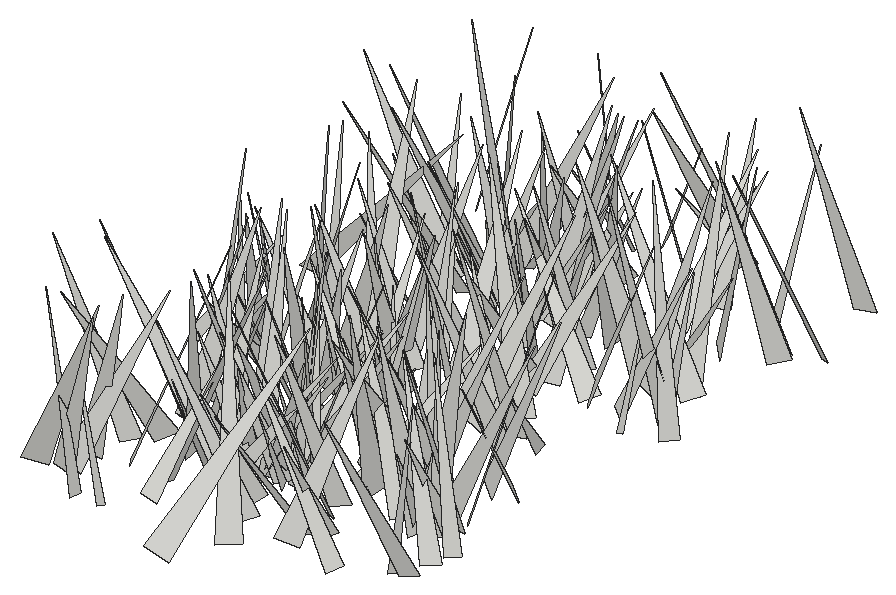
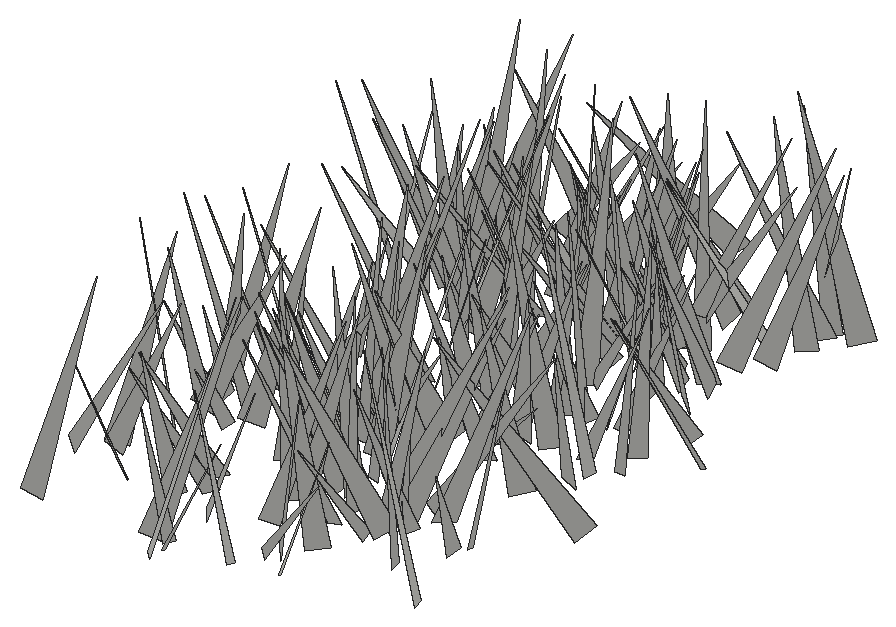
# SketchUp Ruby script. Lengths in inches.
U = 1.inch
M = Sketchup.active_model
def pt(a) = Geom::Point3d.new(a.map { |v| v * U })
def face(e, loops, mat)
  f = e.add_face(loops[0].map { |a| pt(a) })
  loops[1..].each { |l| e.add_face(l.map { |a| pt(a) }).erase! }
  f.material = f.back_material = mat if mat
  f
end
# faces: each face lists its corners as indices into pts; further lists are holes
def faces(e, pts, list, mat = nil) = list.each { |f| face(e, (f[0].is_a?(Array) ? f : [f]).map { |l| l.map { |i| pts[i] } }, mat) }
# xy, xz, yz: faces in a plane at the given z, y or x. An outline is a flat list of corners, or four numbers for a rectangle; further outlines are holes
def ring(l) = l.size == 4 ? [[l[0], l[1]], [l[2], l[1]], [l[2], l[3]], [l[0], l[3]]] : l.each_slice(2).to_a
def flat(e, list, mat, &to3) = list.each { |f| face(e, (f[0].is_a?(Array) ? f : [f]).map { |l| ring(l).map { |u, v| to3.(u, v) } }, mat) }
def xy(e, z, list, mat = nil) = flat(e, list, mat) { |x, y| [x, y, z] }
def xz(e, y, list, mat = nil) = flat(e, list, mat) { |x, z| [x, y, z] }
def yz(e, x, list, mat = nil) = flat(e, list, mat) { |y, z| [x, y, z] }
def lines(e, pts, list) = list.each { |a, b| e.add_line(pt(pts[a]), pt(pts[b])) }
# prism: a flat outline (further loops are holes) pulled along v
def prism(e, loops, v, mat = nil)
  f = face(e, loops, mat); d = Geom::Vector3d.new(v.map { |x| x * U })
  f.pushpull(f.normal.samedirection?(d) ? d.length : -d.length)
end
def box(e, o, s, mat = nil) = prism(e, [[o, [o[0] + s[0], o[1], o[2]], [o[0] + s[0], o[1] + s[1], o[2]], [o[0], o[1] + s[1], o[2]]]], [0, 0, s[2]], mat)
def at(x, y, z, deg = 0) = Geom::Transformation.translation(pt([x, y, z])) * Geom::Transformation.rotation(ORIGIN, Z_AXIS, deg.degrees)
def axes(o, x, y, z) = Geom::Transformation.new([*x, 0, *y, 0, *z, 0, *pt(o).to_a, 1])
def part(name) = M.definitions.add(name)
# library, detail: a bought-in or finely detailed component or shape, given as its bounding box
def library(name, o, s) = part(name).tap { |d| box(d.entities, o, s) }
def detail(e, o, s) = box(e.add_group.entities, o, s)
def put(e, d, t, mat = nil) = e.add_instance(d, t).tap { |i| i.material = mat if mat }
def group(e, t, mat = nil) = e.add_group.tap { |g| g.transformation = t; g.material = mat if mat }.entities
root = M.entities
c1 = part("fur_instance\#9")
p = [[0.8125,0,1.79],[0.67,-0.02,1.48],[0,-0.11,0],[0,0.11,0]]
faces(c1.entities,p,[[0,1,2,3]])
put(root,c1,axes([478.11,318.66,-21.66],[1.0703,-6.74535,2.51722],[-6.58595,-1.94546,-2.41292],[-2.90886,1.9228,6.3893]))
put(root,c1,axes([473.07,330.8,-21.66],[3.04424,4.32162,0.01521],[3.85535,-2.70735,-2.39804],[1.95268,-1.39208,4.71097]))
put(root,c1,axes([478.31,348.03,-21.66],[-4.48023,1.71415,0.10108],[1.53614,4.12726,-1.90446],[0.76734,1.74596,4.4027]))
put(root,c1,axes([478.21,337.2,-21.66],[1.19098,5.93826,0.851],[5.76454,-1.37303,1.51343],[-1.66049,-0.50738,5.86438]))
put(root,c1,axes([476.59,334.39,-21.66],[-1.94792,-5.41513,0.85515],[-5.11405,2.12183,1.78705],[1.97517,0.15336,5.47032]))
put(root,c1,axes([479.69,311.34,-21.66],[-6.30755,-1.0303,0.95825],[-1.23667,6.15876,-1.51833],[0.67114,1.66527,6.20817]))
put(root,c1,axes([479.28,334.33,-21.66],[-4.32688,2.05759,1.06704],[2.30248,4.07514,1.47851],[0.2661,-1.80382,4.55737]))
put(root,c1,axes([477.84,347.04,-21.66],[-4.12038,-2.11418,1.50488],[-1.47976,4.23386,1.89649],[2.13184,-1.14743,4.225]))
put(root,c1,axes([478.76,325.4,-21.66],[4.06044,6.49572,1.60929],[6.19974,-4.35997,1.95581],[-2.5194,-0.26008,7.4065]))
put(root,c1,axes([476.96,332.22,-21.66],[6.03542,-2.39463,0.80521],[-2.12324,-5.9379,-1.74415],[-1.3691,-1.34759,6.25448]))
put(root,c1,axes([475.61,328.35,-21.66],[3.92135,-2.35365,0.03406],[-2.05535,-3.39138,2.27856],[1.14733,1.96892,3.96545]))
put(root,c1,axes([473.56,341.38,-21.66],[6.0984,-4.54505,0.22334],[-3.82324,-4.91501,4.37303],[2.46783,3.61705,6.22291]))
put(root,c1,axes([479.55,320.28,-21.66],[4.2838,-6.03866,0.74714],[-5.20831,-4.11147,-3.36808],[-3.14598,-1.41597,6.59337]))
put(root,c1,axes([475.19,313.07,-21.66],[4.73655,-6.32836,0.37656],[-6.13582,-4.45802,2.25891],[1.59428,1.644,7.57499]))
put(root,c1,axes([481.02,345.5,-21.66],[-7.69272,2.37823,1.5322],[2.71051,7.46743,2.01798],[0.8104,-2.40066,7.79498]))
put(root,c1,axes([481.03,329.86,-21.66],[-5.46466,-2.11839,0.66349],[-2.21236,5.05235,-2.09036],[-0.18243,2.18553,5.47545]))
put(root,c1,axes([482.32,344.96,-21.66],[-2.35699,-6.63901,0.53799],[-6.01099,1.87426,-3.2057],[-2.86948,1.52709,6.27339]))
put(root,c1,axes([476.08,354.2,-21.66],[7.20484,3.15988,1.15153],[3.35999,-6.88107,-2.14053],[-0.14588,-2.42624,7.57051]))
put(root,c1,axes([478.59,323.08,-21.66],[5.94248,2.0649,1.47313],[1.51819,-5.90154,2.14801],[-2.032,1.62942,5.91295]))
put(root,c1,axes([481.06,325.37,-21.66],[-6.67208,0.88571,0.68005],[0.61302,6.34873,-2.25421],[0.93335,2.16166,6.3419]))
put(root,c1,axes([477.25,313.28,-21.66],[0.83878,-6.84447,1.51714],[-6.71971,-0.34936,2.13903],[1.99848,1.69801,6.55552]))
put(root,c1,axes([477.18,315.86,-21.66],[2.07111,-6.85146,1.31632],[-6.80663,-1.68294,1.94991],[1.53132,1.78604,6.88693]))
put(root,c1,axes([484.07,318.57,-21.66],[-5.6206,-6.05261,0.8091],[-5.56666,4.62654,-4.06048],[-2.5102,3.29256,7.1929]))
put(root,c1,axes([479.79,330.34,-21.66],[4.40481,-2.70951,0.82389],[-1.71706,-3.76665,-3.20728],[-2.2521,-2.42766,4.05674]))
put(root,c1,axes([479.56,339.92,-21.66],[-4.86903,5.31705,1.90275],[5.12727,5.21523,-1.45307],[2.36698,-0.35954,7.06166]))
put(root,c1,axes([481.65,311.35,-21.66],[-4.16837,-0.36819,0.02902],[-0.35612,3.91965,-1.4217],[-0.09791,1.41863,3.93569]))
put(root,c1,axes([477.19,313.99,-21.66],[0.42432,7.03314,2.02201],[6.63788,0.48281,-3.07232],[3.08094,-2.00885,6.34082]))
put(root,c1,axes([483.37,320.27,-21.66],[-7.87957,1.88276,1.17896],[2.17634,7.41366,2.70618],[0.44527,-2.91806,7.63603]))
put(root,c1,axes([480.29,323.67,-21.66],[4.99403,0.89918,1.35491],[0.3935,-4.91429,1.81096],[-1.5778,1.62046,4.74018]))
put(root,c1,axes([477.8125,335.72,-21.66],[8.03575,1.73258,0.69022],[1.85682,-7.7181,-2.24381],[-0.17451,-2.34107,7.90825]))
put(root,c1,axes([483.51,348.08,-21.66],[1.68916,7.29229,2.94864],[7.0223,-2.75681,2.79508],[-3.5439,-1.98689,6.94394]))
put(root,c1,axes([479.83,316.42,-21.66],[6.02604,4.35688,0.13616],[4.14402,-5.7981,2.12678],[-1.35204,1.64734,7.12547]))
put(root,c1,axes([479.25,322.59,-21.66],[0.24663,7.62872,2.41582],[7.70784,0.42293,-2.12242],[2.15005,-2.39126,7.33168]))
put(root,c1,axes([483.25,346.38,-21.66],[0.03934,-7.1777,0.79174],[-6.87762,-0.27857,-2.18369],[-2.20103,0.74216,6.83757]))
put(root,c1,axes([480,351.46,-21.66],[6.17791,2.14602,1.95241],[2.61385,-6.11017,-1.55482],[-1.25898,-2.15507,6.35252]))
put(root,c1,axes([484.52,339.01,-21.66],[-3.03964,-3.22245,0.08473],[-2.53096,2.3136,-2.80576],[-1.9964,1.97328,3.42802]))
put(root,c1,axes([484.83,345.3,-21.66],[-3.02685,-7.70536,1.30124],[-7.48247,2.45538,-2.86554],[-2.25353,2.19686,7.76679]))
put(root,c1,axes([482.19,330.73,-21.66],[-7.10447,-2.39928,3.44832],[-3.25719,7.42464,-1.54476],[2.65295,2.69055,7.33783]))
put(root,c1,axes([483.21,323.52,-21.66],[0.69074,-4.72184,2.34998],[-4.89788,-1.45354,-1.48096],[-1.95676,1.97148,4.53648]))
put(root,c1,axes([481.4,322.3,-21.66],[4.67368,1.9817,0.84614],[1.46066,-4.3994,2.23565],[-1.58416,1.79011,4.55767]))
put(root,c1,axes([483.39,321.68,-21.66],[0.65103,4.23875,0.31259],[3.78552,-0.72206,1.9071],[-1.9325,0.01355,3.84107]))
put(root,c1,axes([484.04,334.5625,-21.66],[-0.66678,7.09806,0.59701],[6.83624,0.46921,2.05647],[-2.00116,-0.76214,6.82627]))
put(root,c1,axes([484.17,322.98,-21.66],[-2.33068,3.85921,0.35584],[3.66264,2.05758,1.6744],[-1.26695,-1.15111,4.18592]))
put(root,c1,axes([484.62,326.82,-21.66],[-2.52034,-4.28654,0.32351],[-4.12689,2.30776,-1.57296],[-1.20326,1.06349,4.71724]))
put(root,c1,axes([481.94,330.58,-21.66],[4.14579,-2.60609,2.17076],[-3.31381,-3.84297,1.71517],[-0.72292,2.67047,4.58667]))
put(root,c1,axes([484.58,333.97,-21.66],[-5.48359,2.23586,1.70204],[2.68404,5.27249,1.72124],[0.83185,-2.27324,5.66623]))
put(root,c1,axes([483.26,320.5,-21.66],[-5.22484,3.83291,1.4033],[3.4058,5.3502,-1.93269],[2.24967,0.80218,6.18505]))
put(root,c1,axes([484.76,322.68,-21.66],[-1.35927,-4.19334,1.10265],[-4.18909,0.97193,-1.4678],[-1.11869,1.45561,4.1566]))
put(root,c1,axes([483.79,323.89,-21.66],[-5.87667,-3.9224,1.1719],[-3.54254,5.90008,1.98324],[2.05159,-1.04767,6.78139]))
put(root,c1,axes([486.01,335.86,-21.66],[-1.67581,5.69721,1.32161],[5.39716,0.9769,2.63242],[-2.25291,-1.89755,5.32325]))
put(root,c1,axes([482.33,347.89,-21.66],[3.64505,-0.39812,0.27738],[-0.20845,-3.18305,-1.82936],[-0.43816,-1.79764,3.17779]))
put(root,c1,axes([481.97,319.91,-21.66],[7.49694,-1.26912,1.50095],[-0.87324,-7.45265,-1.93987],[-1.76095,-1.70734,7.35199]))
put(root,c1,axes([483.36,323.23,-21.66],[4.16098,5.56887,0.17793],[5.30628,-4.02846,1.99315],[-1.69922,1.05685,6.65984]))
put(root,c1,axes([485.13,321.75,-21.66],[-7.34828,2.49323,1.09592],[2.03506,7.1224,-2.5582],[1.80991,2.11416,7.32591]))
put(root,c1,axes([481.69,334.51,-21.66],[3.71453,-6.09838,0.78607],[-6.05056,-3.46164,1.73599],[1.09493,1.55972,6.92635]))
put(root,c1,axes([484.27,331.06,-21.66],[6.50516,0.09741,3.11354],[0.81371,-7.01185,-1.48071],[-3.00691,-1.68675,6.33514]))
put(root,c1,axes([481.875,347.5625,-21.66],[2.63596,-3.80697,0.02165],[-3.40971,-2.34911,2.07299],[1.69332,1.196,4.14053]))
put(root,c1,axes([483.36,313.79,-21.66],[-0.37436,5.47936,0.25355],[5.20879,0.43477,-1.70506],[1.71934,-0.12411,5.22075]))
put(root,c1,axes([487.06,355.18,-21.66],[-2.6027,-3.00196,0.39616],[-2.70686,2.07255,-2.07851],[-1.35707,1.62343,3.38609]))
put(root,c1,axes([484.69,356.57,-21.66],[-2.93741,-3.09466,0.01129],[-2.71699,2.58635,2.03327],[1.48156,-1.39259,3.75115]))
put(root,c1,axes([486.47,339.98,-21.66],[1.14957,-5.99203,1.40359],[-5.68779,-1.57972,-2.08556],[-2.35023,0.89221,5.73379]))
put(root,c1,axes([483.59,349.69,-21.66],[3.8069,0.05751,0.20355],[-0.0416,-3.39391,1.73693],[-0.20739,1.73647,3.38805]))
put(root,c1,axes([483.33,330.68,-21.66],[0.81031,-5.69395,0.84212],[-5.55553,-0.55126,1.61834],[1.50543,1.03047,5.51893]))
put(root,c1,axes([486.34,354.46,-21.66],[3.70498,4.05955,2.96614],[3.93602,-4.63444,1.42637],[-3.1282,-1.02317,5.30776]))
put(root,c1,axes([482.92,348.75,-21.66],[6.18283,-3.26103,2.17206],[-3.91127,-5.37775,3.05962],[-0.2327,3.74499,6.28493]))
put(root,c1,axes([486.83,320.23,-21.66],[-7.37463,3.18086,0.67882],[2.84062,7.11825,-2.49505],[1.58417,2.04365,7.63399]))
put(root,c1,axes([486.42,319.71,-21.66],[-4.94323,1.53486,1.76986],[2.06825,4.80019,1.61379],[1.10026,-2.12747,4.91803]))
put(root,c1,axes([483.8,338.05,-21.66],[-0.17372,7.00266,1.70424],[6.95108,0.61311,-1.81067],[1.90374,-1.5996,6.76675]))
put(root,c1,axes([482.94,315.8125,-21.66],[8.11647,0.24258,0.67526],[0.10402,-7.98511,1.61836],[-0.70993,1.60345,7.95719]))
put(root,c1,axes([486.96,336.92,-21.66],[-5.33411,1.7362,0.45715],[1.45522,5.02033,-2.08679],[1.05153,1.85957,5.20696]))
put(root,c1,axes([489.61,315.59,-21.66],[-2.20634,6.02099,1.75888],[5.48729,0.94934,3.63349],[-3.03901,-2.65713,5.28374]))
put(root,c1,axes([484.9,327.28,-21.66],[7.37439,-3.31849,1.28024],[-2.90244,-7.31769,-2.24953],[-2.05603,-1.57231,7.76747]))
put(root,c1,axes([486.43,330.4,-21.66],[-4.56686,4.07542,0.09193],[3.68922,4.19072,-2.51023],[1.73411,1.8173,5.58247]))
put(root,c1,axes([489.04,327.64,-21.66],[-3.06534,4.86368,0.18481],[4.51167,2.75744,2.26433],[-1.82603,-1.35165,5.28436]))
put(root,c1,axes([485.68,320.78,-21.66],[4.75134,-2.11282,0.36953],[-1.90852,-4.57438,-1.61505],[-0.97883,-1.33672,4.94275]))
put(root,c1,axes([487.5,343.29,-21.66],[-5.6893,-5.57398,0.54513],[-5.22917,5.56506,2.3282],[2.00554,-1.30211,7.61688]))
put(root,c1,axes([488.46,330.03,-21.66],[-5.41908,-0.82486,1.13145],[-1.12996,5.24719,-1.58656],[0.82691,1.76453,5.24687]))
put(root,c1,axes([484.43,336.04,-21.66],[3.61715,-5.66391,0.01487],[-5.50634,-3.51236,1.58351],[1.3268,0.86448,6.53117]))
put(root,c1,axes([486.05,348.05,-21.66],[6.38697,0.74513,2.00431],[1.2691,-6.40204,-1.66407],[-1.72101,-1.95564,6.21124]))
put(root,c1,axes([488.38,320.35,-21.66],[2.87814,-5.28951,1.31735],[-4.95416,-3.15966,-1.86304],[-2.27391,0.18887,5.72641]))
put(root,c1,axes([486.94,322.74,-21.66],[5.11337,-4.37567,0.02712],[-4.08728,-4.79107,-2.37351],[-1.56248,-1.78687,6.29758]))
put(root,c1,axes([489.11,341.85,-21.66],[1.07794,-7.21694,3.00432],[-7.53412,-1.768,-1.54384],[-2.08502,2.65746,7.13181]))
put(root,c1,axes([490.07,340.4,-21.66],[-2.15609,-3.98258,0.83043],[-3.73233,1.56246,-2.1972],[-1.61872,1.70208,3.96005]))
put(root,c1,axes([484.88,352.75,-21.66],[3.43044,-6.71204,0.2285],[-6.5076,-3.25868,1.97581],[1.6598,1.09595,7.27431]))
put(root,c1,axes([485.15,324.07,-21.66],[4.61387,-2.10989,0.31356],[-1.93342,-3.82099,2.73855],[0.90102,2.60502,4.2708]))
put(root,c1,axes([488.56,317.84,-21.66],[3.46257,-3.0651,1.27719],[-2.41097,-3.5895,-2.07802],[-2.28326,-0.85797,4.13111]))
put(root,c1,axes([489.51,348.25,-21.66],[0.21483,-6.37799,2.26736],[-6.52313,-0.80094,-1.63496],[-1.80789,2.13204,6.16862]))
put(root,c1,axes([488.94,336.27,-21.66],[-6.13074,4.86156,0.06985],[4.48302,5.69573,-2.94734],[1.88206,2.26926,7.24803]))
put(root,c1,axes([487.48,333.01,-21.66],[7.10031,-2.91459,1.55919],[-2.29482,-7.00551,-2.64516],[-2.37902,-1.94118,7.20502]))
put(root,c1,axes([486.01,349.71,-21.66],[1.82211,6.46965,0.85286],[6.26515,-1.48669,-2.10749],[1.8253,-1.35544,6.38239]))
put(root,c1,axes([489.1875,320.28,-21.66],[2.9038,6.51052,1.10748],[6.2299,-3.10193,1.9005],[-2.1913,-0.1914,6.87074]))
put(root,c1,axes([487.54,344.11,-21.66],[-3.32814,-6.39102,1.50803],[-6.07577,3.63841,2.01068],[2.49085,0.3356,6.91945]))
put(root,c1,axes([486.22,340.9,-21.66],[3.6811,-6.05089,2.6185],[-6.53456,-2.94932,2.37094],[0.87715,3.42178,6.67401]))
put(root,c1,axes([490.53,312.37,-21.66],[-7.32021,3.8589,0.48336],[3.73123,7.2592,-1.44642],[1.09666,1.05977,8.14767]))
put(root,c1,axes([491.01,322.1,-21.66],[-4.07281,-4.5818,0.7427],[-4.55178,3.7491,-1.83244],[-0.90871,1.75604,5.85003]))
put(root,c1,axes([489.72,332.18,-21.66],[-6.30964,2.41528,1.06239],[1.96226,6.1361,-2.29599],[1.76402,1.81341,6.35402]))
put(root,c1,axes([490.02,320.78,-21.66],[-5.70534,2.42628,0.74712],[2.22137,5.6608,-1.42016],[1.22905,1.03174,6.03498]))
put(root,c1,axes([488.65,319.97,-21.66],[-3.02452,-1.82217,1.01563],[-1.34667,3.07159,1.50047],[1.5932,-0.86291,3.19635]))
put(root,c1,axes([489.21,351.96,-21.66],[4.98513,-4.06782,0.78587],[-3.3159,-4.65458,-3.05875],[-2.48386,-1.95039,5.66063]))
put(root,c1,axes([490.43,328.35,-21.66],[-4.5545,1.12209,0.15618],[1.0267,4.36161,-1.39615],[0.47894,1.3207,4.4781]))
put(root,c1,axes([492.1,332.26,-21.66],[-6.74391,-2.32387,0.77011],[-2.44649,6.31426,-2.37034],[-0.09,2.49068,6.72772]))
put(root,c1,axes([488.5,345.33,-21.66],[6.0321,-2.57805,3.10449],[-3.62742,-5.91038,2.14001],[-1.76807,3.33038,6.20104]))
put(root,c1,axes([487.1,346.42,-21.66],[1.41766,-6.83451,0.48866],[-6.53171,-1.19719,2.20513],[2.07029,0.90294,6.62252]))
put(root,c1,axes([488.29,346.19,-21.66],[6.56769,-0.93589,1.93904],[-1.50422,-6.44796,1.98276],[-1.54048,2.30611,6.3308]))
put(root,c1,axes([486.68,319.97,-21.66],[3.67258,4.04026,0.63824],[3.75616,-2.99162,-2.6759],[1.61937,-2.22383,4.75932]))
put(root,c1,axes([485.88,317.94,-21.66],[4.06376,5.39951,0.02576],[4.83357,-3.62337,-3.0294],[2.40665,-1.8401,6.04083]))
put(root,c1,axes([487.64,320.32,-21.66],[2.89446,-5.47209,0.08006],[-5.31049,-2.7865,1.53693],[1.32243,0.78724,5.99662]))
put(root,c1,axes([487.96,308.73,-21.66],[-4.06981,7.2471,0.38585],[5.9474,3.58401,-4.58433],[4.15906,1.9665,6.9331]))
put(root,c1,axes([493.17,318.85,-21.66],[-4.54236,-5.48641,0.31776],[-5.31376,4.27953,-2.06985],[-1.40202,1.55551,6.81539]))
put(root,c1,axes([487.82,357.32,-21.66],[5.19096,1.17327,0.15724],[1.14991,-4.82989,-1.92283],[0.28108,-1.90867,4.96239]))
put(root,c1,axes([489.51,321.9,-21.66],[6.5233,2.37968,3.04495],[3.30026,-6.53866,-1.96019],[-2.01069,-3.01183,6.66138]))
put(root,c1,axes([489.37,320.36,-21.66],[5.91646,3.40669,0.5347],[3.12979,-5.75065,2.00759],[-1.44773,1.49011,6.52531]))
put(root,c1,axes([487.25,321.8,-21.66],[2.23337,6.49328,0.05356],[5.9184,-2.0122,-2.84202],[2.67172,-0.9705,6.25089]))
put(root,c1,axes([492.64,353.61,-21.66],[-4.27144,-3.27285,0.83505],[-3.36103,3.98484,-1.57435],[-0.33515,1.75031,5.14569]))
put(root,c1,axes([492.19,318.79,-21.66],[0.25275,3.74041,1.98428],[3.79537,-1.08135,1.55493],[-1.87703,-1.68284,3.41127]))
put(root,c1,axes([487.97,344.26,-21.66],[4.83025,3.81866,0.07193],[3.65702,-4.5907,-1.86288],[1.10161,-1.50398,5.86882]))
put(root,c1,axes([490.22,345.01,-21.66],[5.08436,-3.96797,0.13679],[-3.71243,-4.83007,-2.12193],[-1.40762,-1.5937,6.0904]))
put(root,c1,axes([489.875,344.37,-21.66],[7.02888,1.27959,1.54515],[0.73768,-6.88381,2.34499],[-1.86566,2.099,6.7486]))
put(root,c1,axes([493.41,316.24,-21.66],[-0.91918,-4.72146,0.08029],[-4.18667,0.777,-2.23865],[-2.18412,0.49761,4.25741]))
put(root,c1,axes([489.04,345.02,-21.66],[-0.29614,5.30233,1.4786],[4.87042,0.94241,-2.40408],[2.56516,-1.17721,4.73528]))
put(root,c1,axes([492,358.52,-21.66],[-3.24466,-1.65637,0.06319],[-1.44148,2.88818,1.68993],[0.81834,-1.47993,3.2273]))
put(root,c1,axes([488.17,322.26,-21.66],[4.70359,-4.43483,0.77561],[-4.1988,-3.91632,3.07011],[1.62462,2.71804,5.6891]))
put(root,c1,axes([493.7,324.32,-21.66],[-0.77186,4.35622,1.72795],[4.2436,-0.09339,2.13104],[-1.98854,-1.8902,3.87699]))
put(root,c1,axes([492.8,320.14,-21.66],[2.20766,-6.15742,1.48059],[-5.96151,-2.54967,-1.71445],[-2.13691,0.75174,6.31254]))
put(root,c1,axes([492.27,359.59,-21.66],[-6.0329,-5.73941,0.68236],[-5.34499,5.91535,2.49841],[2.19943,-1.36753,7.94322]))
put(root,c1,axes([492.41,339.16,-21.66],[3.27442,-5.47757,0.11686],[-5.10679,-3.10069,-2.24625],[-1.98447,-1.05885,5.97327]))
put(root,c1,axes([491.02,340.89,-21.66],[-2.08812,-6.42397,1.05341],[-6.15561,2.30841,1.87538],[2.11792,0.37569,6.48927]))
put(root,c1,axes([492.36,322.82,-21.66],[3.62911,6.60842,0.2466],[6.35712,-3.56375,1.94657],[-1.82181,0.72867,7.28371]))
put(root,c1,axes([489.92,349.03,-21.66],[-0.39765,-7.51588,0.89638],[-7.02687,0.7002,2.75371],[2.81337,0.68655,7.00455]))
put(root,c1,axes([493.85,342.28,-21.66],[-0.12405,-5.8754,2.10648],[-6.00776,-0.4589,-1.63376],[-1.69244,2.05962,5.64504]))
put(root,c1,axes([490.99,327.69,-21.66],[5.45875,-2.61976,0.1584],[-2.41646,-5.15945,-2.05595],[-1.02417,-1.78972,5.6951]))
put(root,c1,axes([496.28,339.57,-21.66],[-3.37764,5.82202,0.02709],[5.22944,3.02002,2.9728],[-2.55923,-1.51283,6.03878]))
put(root,c1,axes([490.9,324.6,-21.66],[1.63148,3.88333,0.8996],[3.80186,-1.22375,-1.61232],[1.19808,-1.40479,3.89132]))
put(root,c1,axes([494.57,335.22,-21.66],[-3.07753,7.46975,2.03134],[7.70521,2.74591,1.57617],[-0.74375,-2.46119,7.92363]))
put(root,c1,axes([494.6,333.22,-21.66],[-1.73609,5.26171,0.91511],[5.1615,1.40586,1.70864],[-1.37182,-1.3693,5.27069]))
put(root,c1,axes([491.27,345.11,-21.66],[5.10289,-1.83511,1.25864],[-2.13691,-4.91957,1.49087],[-0.62081,1.84972,5.21387]))
put(root,c1,axes([494.61,326.91,-21.66],[1.00631,5.78428,1.17144],[5.41169,-1.37849,2.15781],[-2.35451,-0.6962,5.46025]))
put(root,c1,axes([494.09,328.02,-21.66],[-5.79035,-4.99721,0.36352],[-4.82955,5.71454,1.62848],[1.33407,-1.00217,7.47317]))
put(root,c1,axes([493.46,357.75,-21.66],[3.75973,-6.87339,0.18092],[-6.4988,-3.61971,-2.46477],[-2.2454,-1.03249,7.43666]))
put(root,c1,axes([493.24,322.82,-21.66],[-5.97447,-2.65496,2.2585],[-2.10106,6.3191,1.8704],[2.78122,-0.92951,6.26456]))
put(root,c1,axes([497.41,313.9,-21.66],[-2.18408,5.95276,0.46734],[5.01759,1.55993,3.57972],[-3.2369,-1.59851,5.23366]))
put(root,c1,axes([493.32,339.6,-21.66],[-2.78361,3.37072,1.19614],[3.02117,3.0272,-1.49988],[1.91443,0.12385,4.10617]))
put(root,c1,axes([495.82,333.25,-21.66],[-1.13695,-6.80591,1.9758],[-6.92615,0.64332,-1.76957],[-1.50086,2.18691,6.66945]))
put(root,c1,axes([492.3,357.58,-21.66],[1.15805,-3.96128,0.43832],[-3.70743,-0.90324,1.63219],[1.46246,0.84697,3.79062]))
put(root,c1,axes([493.23,345.64,-21.66],[5.19652,-2.78136,0.42044],[-2.54268,-5.02221,-1.79688],[-1.20313,-1.39929,5.61347]))
put(root,c1,axes([494.23,326.23,-21.66],[6.48177,-5.01878,0.45242],[-4.24735,-5.8379,-3.90962],[-2.71162,-2.85253,7.2053]))
put(root,c1,axes([493.49,322.65,-21.66],[7.48346,-2.4752,1.75576],[-1.96533,-7.51292,-2.21472],[-2.31232,-1.62508,7.56464]))
put(root,c1,axes([494.61,317.04,-21.66],[2.5877,-3.76016,0.15432],[-3.53923,-2.49522,-1.45139],[-1.27925,-0.70276,4.32764]))
put(root,c1,axes([496.56,321.24,-21.66],[-3.37701,5.49526,1.43426],[5.6473,3.0721,1.52623],[-0.60248,-2.00587,6.26679]))
put(root,c1,axes([496.47,331.17,-21.66],[-7.7703,-1.5883,1.42664],[-1.2052,7.70803,2.01725],[1.76224,-1.7318,7.67014]))
put(root,c1,axes([493.1,314.6875,-21.66],[-3.36255,6.42423,2.20976],[5.77924,4.00105,-2.8377],[3.57129,-0.42595,6.67271]))
put(root,c1,axes([495.81,326.25,-21.66],[2.24091,-5.47361,0.67385],[-5.23088,-2.33999,-1.61199],[-1.7471,-0.01469,5.69066]))
put(root,c1,axes([492.25,322.5,-21.66],[0.90469,6.24799,0.05202],[5.52251,-0.775,-2.9597],[2.92267,-0.46962,5.57638]))
put(root,c1,axes([492.68,332.78,-21.66],[1.48421,7.77893,1.22221],[7.56365,-1.06243,-2.42301],[2.19017,-1.60247,7.53948]))
put(root,c1,axes([492.47,338.4,-21.66],[1.86343,6.88556,0.79652],[6.51007,-1.45535,-2.64927],[2.37997,-1.41024,6.62304]))
put(root,c1,axes([495.49,352.93,-21.66],[-4.4871,3.83069,1.41429],[3.5666,4.69982,-1.41404],[1.98841,0.2144,5.72789]))
put(root,c1,axes([494.17,351.27,-21.66],[-1.05033,5.0969,0.69056],[4.61293,1.24522,-2.17458],[2.27512,-0.17172,4.72788]))
put(root,c1,axes([494.95,349.52,-21.66],[-2.16647,5.60636,0.16983],[5.26617,2.09582,-2.00715],[1.93067,0.57445,5.66535]))
put(root,c1,axes([497.54,343.25,-21.66],[2.58278,-6.81445,2.81399],[-6.72051,-3.40212,-2.07037],[-3.03151,1.73634,6.98721]))
put(root,c1,axes([494.23,326.54,-21.66],[3.12045,6.97557,0.92804],[6.87353,-2.80376,-2.03727],[1.5081,-1.6545,7.36514]))
put(root,c1,axes([501.0625,343.41,-21.66],[-3.57057,6.8988,1.02898],[6.50769,2.8788,3.28081],[-2.51043,-2.34953,7.04122]))
put(root,c1,axes([496.09,325.26,-21.66],[2.2039,-6.87435,1.74953],[-7.02125,-1.85328,1.56272],[1.00974,2.1174,7.04782]))
put(root,c1,axes([495.41,325.48,-21.66],[3.73995,-4.97965,1.07609],[-4.97131,-3.27521,2.12161],[1.114,2.10195,5.85517]))
put(root,c1,axes([499.59,320.73,-21.66],[-6.16922,0.32467,1.04524],[-0.06119,5.87189,-2.18505],[1.09279,2.16166,5.77844]))
put(root,c1,axes([497.82,332.89,-21.66],[3.38324,-1.277,0.34003],[-0.90165,-2.91389,-1.97203],[-0.96612,-1.75247,3.03119]))
put(root,c1,axes([498.55,320.6875,-21.66],[6.46231,-4.31648,2.52967],[-3.92803,-6.93665,-1.8017],[-3.09867,-0.20881,7.55958]))
put(root,c1,axes([500.3,322.1875,-21.66],[-2.82559,-5.19892,1.36333],[-5.31081,2.46391,-1.61114],[-0.82624,1.9421,5.69358]))
put(root,c1,axes([496.22,339.52,-21.66],[5.98331,3.57339,0.75673],[3.63565,-5.68637,-1.89446],[0.35186,-2.00943,6.70672]))
put(root,c1,axes([498.28,320.99,-21.66],[4.1039,-1.37964,0.4984],[-1.03776,-3.77714,-1.91052],[-1.03675,-1.68037,3.88527]))
put(root,c1,axes([501.5,317.89,-21.66],[-1.94953,6.2532,0.70862],[6.08536,1.68405,1.8809],[-1.60411,-1.2111,6.27419]))
put(root,c1,axes([499.68,352.68,-21.66],[2.78013,5.13783,0.11647],[4.85085,-2.66723,1.86951],[-1.69707,0.79284,5.53456]))
put(root,c1,axes([502.04,350.7,-21.66],[-0.7555,-5.85213,2.53673],[-5.87032,-0.36099,-2.58111],[-2.49433,2.62211,5.30623]))
put(root,c1,axes([500.16,323.125,-21.66],[5.94606,5.36025,0.59468],[4.2161,-5.17199,4.4628],[-3.36309,2.9933,6.64615]))
put(root,c1,axes([500.6,343.68,-21.66],[0.70826,8.01559,0.32411],[7.89046,-0.75477,1.42384],[-1.44754,-0.19233,7.91985]))
put(root,c1,axes([500.39,315.71,-21.66],[-4.99347,0.21503,1.45697],[-0.36457,4.80955,-1.95935],[1.42691,1.98134,4.59803]))
put(root,c1,axes([500.3,337.35,-21.66],[1.53322,3.39,0.04746],[3.12816,-1.43461,1.41479],[-1.30727,0.54307,3.44111]))
put(root,c1,axes([501.91,319.47,-21.66],[-0.60049,6.11637,0.8715],[5.86899,0.29123,2.00004],[-1.92986,-1.0175,5.81123]))
put(root,c1,axes([501.3,316.12,-21.66],[1.05272,-6.58483,0.46236],[-6.33643,-1.13928,-1.79827],[-1.85027,0.15508,6.42141]))
put(root,c1,axes([498.26,342.42,-21.66],[2.40948,7.1196,1.80641],[7.28749,-2.07931,-1.52526],[0.91887,-2.17835,7.35989]))
put(root,c1,axes([500.02,321.7,-21.66],[4.14247,-2.36814,0.94959],[-1.79033,-3.98803,-2.13546],[-1.81783,-1.46881,4.26707]))
put(root,c1,axes([502,339.81,-21.66],[-1.47229,-7.46087,2.3597],[-7.72207,0.99683,-1.66627],[-1.2659,2.59656,7.41996]))
put(root,c1,axes([498.41,344.35,-21.66],[4.05513,-1.76427,0.28786],[-1.75227,-3.78191,1.50543],[0.35366,1.49134,4.15818]))
put(root,c1,axes([500.63,341.57,-21.66],[-3.9364,0.91485,1.26316],[0.41585,3.92071,-1.54367],[1.50319,1.31107,3.73488]))
put(root,c1,axes([498.67,348.79,-21.66],[5.37674,4.78999,2.15375],[5.23773,-5.117,-1.69543],[-0.38579,-2.71372,6.99849]))
put(root,c1,axes([503.14,338.53,-21.66],[-7.7657,1.30292,0.44128],[1.14319,7.51969,-2.08465],[0.76515,1.98873,7.59328]))
put(root,c1,axes([499.99,327.85,-21.66],[-3.50557,-5.51536,0.11612],[-4.95597,3.20905,2.80393],[2.42302,-1.41579,5.90306]))
put(root,c1,axes([502.38,358.1,-21.66],[0.14854,-7.36709,1.66817],[-7.40985,-0.46607,-1.39849],[-1.46661,1.60862,7.23466]))
put(root,c1,axes([504.28,351.91,-21.66],[-3.99389,-5.07881,0.29207],[-4.86869,3.70838,-2.09153],[-1.47493,1.51142,6.11318]))
put(root,c1,axes([502.29,350.06,-21.66],[3.31279,-6.01066,2.01721],[-5.81791,-3.7865,-1.72802],[-2.51972,0.84034,6.64203]))
put(root,c1,axes([498.39,327.23,-21.66],[4.54413,5.8348,1.67226],[5.93472,-3.83302,-2.75273],[1.27295,-2.95864,6.86415]))
put(root,c1,axes([498.81,339.12,-21.66],[3.86219,5.07234,0.99731],[5.04282,-3.42294,-2.11973],[1.1372,-2.04809,6.01264]))
put(root,c1,axes([498.79,322.66,-21.66],[5.79439,-3.93356,1.43708],[-4.17619,-5.2444,2.48372],[0.31237,2.85246,6.54821]))
